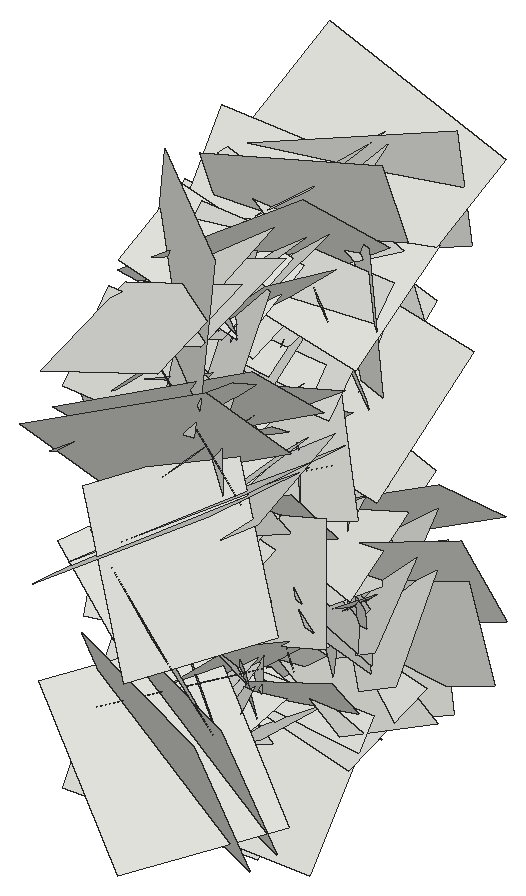
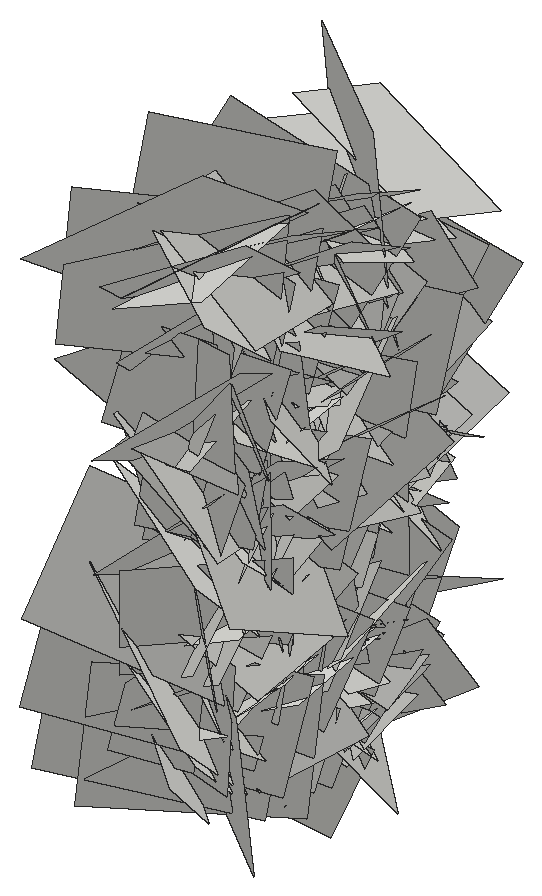
# SketchUp Ruby script. Lengths in inches.
U = 1.inch
M = Sketchup.active_model
def pt(a) = Geom::Point3d.new(a.map { |v| v * U })
def face(e, loops, mat)
  f = e.add_face(loops[0].map { |a| pt(a) })
  loops[1..].each { |l| e.add_face(l.map { |a| pt(a) }).erase! }
  f.material = f.back_material = mat if mat
  f
end
# faces: each face lists its corners as indices into pts; further lists are holes
def faces(e, pts, list, mat = nil) = list.each { |f| face(e, (f[0].is_a?(Array) ? f : [f]).map { |l| l.map { |i| pts[i] } }, mat) }
# xy, xz, yz: faces in a plane at the given z, y or x. An outline is a flat list of corners, or four numbers for a rectangle; further outlines are holes
def ring(l) = l.size == 4 ? [[l[0], l[1]], [l[2], l[1]], [l[2], l[3]], [l[0], l[3]]] : l.each_slice(2).to_a
def flat(e, list, mat, &to3) = list.each { |f| face(e, (f[0].is_a?(Array) ? f : [f]).map { |l| ring(l).map { |u, v| to3.(u, v) } }, mat) }
def xy(e, z, list, mat = nil) = flat(e, list, mat) { |x, y| [x, y, z] }
def xz(e, y, list, mat = nil) = flat(e, list, mat) { |x, z| [x, y, z] }
def yz(e, x, list, mat = nil) = flat(e, list, mat) { |y, z| [x, y, z] }
def lines(e, pts, list) = list.each { |a, b| e.add_line(pt(pts[a]), pt(pts[b])) }
# prism: a flat outline (further loops are holes) pulled along v
def prism(e, loops, v, mat = nil)
  f = face(e, loops, mat); d = Geom::Vector3d.new(v.map { |x| x * U })
  f.pushpull(f.normal.samedirection?(d) ? d.length : -d.length)
end
def box(e, o, s, mat = nil) = prism(e, [[o, [o[0] + s[0], o[1], o[2]], [o[0] + s[0], o[1] + s[1], o[2]], [o[0], o[1] + s[1], o[2]]]], [0, 0, s[2]], mat)
def at(x, y, z, deg = 0) = Geom::Transformation.translation(pt([x, y, z])) * Geom::Transformation.rotation(ORIGIN, Z_AXIS, deg.degrees)
def axes(o, x, y, z) = Geom::Transformation.new([*x, 0, *y, 0, *z, 0, *pt(o).to_a, 1])
def part(name) = M.definitions.add(name)
# library, detail: a bought-in or finely detailed component or shape, given as its bounding box
def library(name, o, s) = part(name).tap { |d| box(d.entities, o, s) }
def detail(e, o, s) = box(e.add_group.entities, o, s)
def put(e, d, t, mat = nil) = e.add_instance(d, t).tap { |i| i.material = mat if mat }
def group(e, t, mat = nil) = e.add_group.tap { |g| g.transformation = t; g.material = mat if mat }.entities
root = M.entities
c1 = part("Component\#6")
p = [[0.01,0,0],[0,3.24,4.54],[4.32,3.24,4.54],[4.33,0,0]]
faces(c1.entities,p,[[0,1,2,3]])
put(root,c1,axes([424.49,133.2,0.29],[0.16868,0.00753,1.30134],[0.16064,1.302,-0.02607],[-1.37005,0.15359,0.15716]))
put(root,c1,axes([420.52,134.57,7.51],[-0.06425,-0.0713,-0.65597],[0.02618,-0.65852,0.06929],[0.69893,0.01811,-0.0629]))
put(root,c1,axes([424.49,128.52,17.74],[-0.08604,0.43028,-0.81229],[-0.04293,-0.81633,-0.42838],[-0.97342,-0.00203,0.0907]))
put(root,c1,axes([420.52,132.11,13.83],[-0.12823,-0.67114,-0.46171],[-0.10246,-0.45164,0.68184],[0.85739,-0.15435,0.01243]))
put(root,c1,axes([424.49,133.79,15.82],[-0.11741,-0.82822,-0.37202],[-0.00882,-0.37384,0.83474],[-0.96237,0.10447,0.03774]))
put(root,c1,axes([420.52,131.53,3.64],[-0.03356,0.34972,-0.55611],[0.01458,-0.55628,-0.35061],[0.69619,0.02851,-0.01946]))
put(root,c1,axes([420.52,130.57,14.69],[-0.08088,0.56373,-0.36339],[0.06437,-0.35843,-0.56878],[0.70803,0.09698,0.0102]))
put(root,c1,axes([424.49,130.125,12.36],[0.14413,1.23778,0.56401],[0.30073,0.52855,-1.22835],[-1.41013,0.23923,-0.20431]))
put(root,c1,axes([424.49,129.28,18.375],[-0.15104,-0.37703,-0.77667],[0.00911,-0.78776,0.38083],[-0.9151,0.05438,0.13199]))
put(root,c1,axes([424.49,132.6,22.9],[-0.05818,0.99288,0.05669],[0.07779,0.06066,-0.99145],[-1.05129,-0.05046,-0.07649]))
put(root,c1,axes([420.52,133.3125,17.59],[0.01529,0.27468,0.5349],[0.08187,0.52978,-0.27413],[0.6321,-0.07526,0.02257]))
put(root,c1,axes([420.52,129.84,16.13],[0.05288,0.68465,0.04631],[-0.09068,0.05228,-0.68068],[0.72171,-0.04359,-0.08892]))
put(root,c1,axes([424.49,129.45,15.69],[0.00555,0.72683,0.86308],[0.19522,0.85097,-0.71774],[-1.18002,0.1442,-0.11468]))
put(root,c1,axes([420.52,129.41,10.95],[-0.18775,-0.48629,-0.69123],[0.00245,-0.70652,0.49646],[0.89586,-0.09998,-0.14623]))
put(root,c1,axes([420.52,132.63,6.14],[-0.10731,0.87556,-0.00554],[-0.12201,-0.01884,-0.87366],[0.92006,0.09962,-0.1165]))
put(root,c1,axes([424.49,133.96,12.5],[-0.03937,0.24323,0.81298],[-0.12274,0.80469,-0.24604],[-0.89109,-0.12158,-0.00203]))
put(root,c1,axes([424.49,127.6,6.32],[-0.09105,0.77875,-0.27248],[-0.08108,-0.28029,-0.77696],[-0.87078,-0.05533,0.10084]))
put(root,c1,axes([424.49,133.1,9.3125],[0.02086,0.87239,-0.16813],[-0.14049,-0.16341,-0.8634],[-0.93122,0.04419,0.12649]))
put(root,c1,axes([424.49,131.05,1.96],[0.03915,-1.05631,0.36623],[0.17317,0.36759,1.04378],[-1.17236,0.01903,0.16641]))
put(root,c1,axes([420.52,133.88,6.93],[-0.12434,-0.60409,0.41763],[0.12699,0.40152,0.61444],[0.76804,-0.16419,-0.03398]))
put(root,c1,axes([424.49,136.93,7.59],[0.11136,0.24127,-0.97313],[-0.07388,-0.97433,-0.24909],[-1.06018,0.09324,-0.08486]))
put(root,c1,axes([420.52,130.03,2.94],[-0.11679,-0.3481,0.76621],[-0.04914,0.77408,0.34502],[0.89071,-0.00294,0.1195]))
put(root,c1,axes([420.52,129.23,5.41],[-0.17398,-0.60139,0.60701],[0.02487,0.6147,0.61536],[0.9054,-0.13245,0.09973]))
put(root,c1,axes([424.49,132.5,3.06],[0.12033,-0.77552,-0.96336],[0.26418,-0.93322,0.78062],[-1.28404,-0.26468,0.07033]))
put(root,c1,axes([420.52,129.18,10.77],[0.08644,0.04023,-0.60323],[0.06997,-0.60565,-0.03147],[0.63702,0.06107,0.08531]))
put(root,c1,axes([424.49,132.55,10.48],[0.11298,-1.07137,-0.22101],[0.09706,-0.21254,1.07447],[-1.1555,-0.12261,0.06864]))
put(root,c1,axes([420.52,128.34,18.92],[0.04874,0.38349,0.62334],[-0.06251,0.62448,-0.37984],[0.77325,0.02631,-0.07]))
put(root,c1,axes([420.52,129.8,15.91],[0.05085,-0.71724,0.33006],[-0.13843,0.31891,0.71198],[0.82538,0.09767,0.09907]))
put(root,c1,axes([424.49,127.86,19.19],[0.25173,1.01088,0.57921],[0.04385,0.58343,-1.03521],[-1.23418,0.22691,0.08136]))
put(root,c1,axes([424.49,127.34,21.1],[0.03089,0.79811,0.32897],[-0.11706,0.3299,-0.79059],[-0.90753,-0.01539,0.11317]))
put(root,c1,axes([420.52,133.42,16.97],[-0.14677,0.94615,0.46149],[-0.22557,0.4307,-0.94687],[1.09283,0.21597,-0.13346]))
put(root,c1,axes([420.52,133.96,6.46],[-0.0893,0.11056,0.97068],[-0.19494,0.95507,-0.12474],[1.01706,0.19277,0.06132]))
put(root,c1,axes([424.49,136.53,11.26],[0.01536,-0.64622,-0.54667],[-0.11065,-0.54394,0.64022],[-0.89037,0.05645,-0.089]))
put(root,c1,axes([420.52,131.99,-0.9375],[0.0225,-0.54484,0.50649],[-0.02225,0.50605,0.54525],[0.78821,0.02984,0.00093]))
put(root,c1,axes([424.49,127.95,5.4],[-0.05879,0.74539,0.22064],[-0.10629,0.21249,-0.74307],[-0.81711,-0.08127,0.08079]))
put(root,c1,axes([420.52,125.86,8.82],[0.02658,0.53015,0.39509],[0.11889,0.38623,-0.52538],[0.69069,-0.08688,0.07523]))
put(root,c1,axes([420.52,131.86,3.01],[0.01467,-0.55248,-0.51034],[-0.00827,-0.51051,0.55244],[0.7972,0.00487,0.01512]))
put(root,c1,axes([420.52,136.82,15.87],[-0.16772,-0.74319,-0.48228],[0.03783,-0.49486,0.75087],[0.93836,-0.11289,-0.11647]))
put(root,c1,axes([424.49,125.93,11.7],[-0.16945,0.67455,-0.05214],[-0.09647,-0.07453,-0.68517],[-0.71064,-0.15073,0.10544]))
put(root,c1,axes([424.49,127.92,4.7],[-0.092,0.70183,0.2556],[-0.07294,0.24871,-0.70628],[-0.78837,-0.10491,0.03552]))
put(root,c1,axes([424.49,128.53,16.93],[0.30517,1.08519,-0.55956],[0.1011,-0.59314,-1.10124],[-1.29027,0.21019,-0.21864]))
put(root,c1,axes([420.52,137.37,4.77],[-0.01509,-0.67708,-0.46908],[-0.05072,-0.46768,0.67651],[0.87164,-0.03894,0.03124]))
put(root,c1,axes([424.49,133.14,16.06],[0.03738,-0.31853,0.81486],[-0.04959,0.81367,0.32009],[-0.92608,-0.05642,0.01575]))
put(root,c1,axes([424.49,133.58,20.74],[0.06025,0.71815,0.57437],[0.00066,0.57544,-0.71955],[-0.97476,0.04478,0.03501]))
put(root,c1,axes([424.49,131.35,15.19],[-0.02447,0.82058,-0.14823],[-0.01236,-0.14859,-0.82075],[-0.8838,-0.02064,0.01558]))
put(root,c1,axes([420.52,130.01,4.69],[0.05447,0.12092,0.77662],[-0.06993,0.77619,-0.11649],[0.83019,0.05744,-0.06077]))
put(root,c1,axes([424.49,135.14,15.06],[0.15738,0.18416,-1.10832],[0.16264,-1.1108,-0.16402],[-1.17977,-0.12857,-0.17046]))
put(root,c1,axes([424.49,133.07,14.74],[0.12706,0.28525,0.91315],[-0.02767,0.92092,-0.28425],[-1.01369,0.01061,0.12222]))
put(root,c1,axes([424.49,132.96,18.89],[0.10145,-0.91774,-0.17179],[-0.02227,-0.17476,0.92192],[-0.98945,-0.09016,-0.03837]))
put(root,c1,axes([420.52,135.65,2.32],[-0.1935,-1.06071,0.09437],[-0.13048,0.11613,1.0671],[1.12123,-0.16954,0.14047]))
put(root,c1,axes([420.52,136.42,13.64],[0.14309,-0.55174,0.41683],[-0.03038,0.41987,0.56505],[0.73236,0.12522,-0.058]))
put(root,c1,axes([424.49,137.27,19.36],[0.1763,0.15017,-0.9005],[-0.15684,-0.89878,-0.17721],[-0.95491,0.17535,-0.13715]))
put(root,c1,axes([424.49,130.2,1.79],[0.1042,-0.77086,0.73803],[0.17604,0.74317,0.75412],[-1.11745,0.04519,0.18762]))
put(root,c1,axes([424.49,136.01,11.51],[-0.06598,-0.27091,0.62957],[-0.16839,0.62065,0.25136],[-0.70672,-0.12259,-0.11867]))
put(root,c1,axes([420.52,133.51,8.98],[-0.15319,0.47062,-0.90401],[-0.09722,-0.91536,-0.46187],[1.07594,-0.0157,-0.17044]))
put(root,c1,axes([424.49,126.24,11.02],[-0.17433,0.41563,0.4957],[-0.04437,0.50356,-0.43611],[-0.68427,-0.13854,-0.09801]))
put(root,c1,axes([420.52,132.67,11.61],[-0.16439,-1.14375,-0.17253],[-0.24163,-0.14044,1.13591],[1.20204,-0.18465,0.20475]))
put(root,c1,axes([424.49,132.67,11.61],[0.16439,-1.14375,-0.17253],[0.24163,-0.14044,1.13591],[-1.20204,-0.18465,0.20475]))
put(root,c1,axes([420.52,126.24,11.02],[0.17433,0.41563,0.4957],[0.04437,0.50356,-0.43611],[0.68427,-0.13854,-0.09801]))
put(root,c1,axes([424.49,133.51,8.98],[0.15319,0.47062,-0.90401],[0.09722,-0.91536,-0.46187],[-1.07594,-0.0157,-0.17044]))
put(root,c1,axes([420.52,136.01,11.51],[0.06598,-0.27091,0.62957],[0.16839,0.62065,0.25136],[0.70672,-0.12259,-0.11867]))
put(root,c1,axes([420.52,130.2,1.79],[-0.1042,-0.77086,0.73803],[-0.17604,0.74317,0.75412],[1.11745,0.04519,0.18762]))
put(root,c1,axes([420.52,137.27,19.36],[-0.1763,0.15017,-0.9005],[0.15684,-0.89878,-0.17721],[0.95491,0.17535,-0.13715]))
put(root,c1,axes([424.49,136.42,13.64],[-0.14309,-0.55174,0.41683],[0.03038,0.41987,0.56505],[-0.73236,0.12522,-0.058]))
put(root,c1,axes([424.49,135.65,2.32],[0.1935,-1.06071,0.09437],[0.13048,0.11613,1.0671],[-1.12123,-0.16954,0.14047]))
put(root,c1,axes([420.52,132.96,18.89],[-0.10145,-0.91774,-0.17179],[0.02227,-0.17476,0.92192],[0.98945,-0.09016,-0.03837]))
put(root,c1,axes([420.52,133.07,14.74],[-0.12706,0.28525,0.91315],[0.02767,0.92092,-0.28425],[1.01369,0.01061,0.12222]))
put(root,c1,axes([420.52,135.14,15.06],[-0.15738,0.18416,-1.10832],[-0.16264,-1.1108,-0.16402],[1.17977,-0.12857,-0.17046]))
put(root,c1,axes([424.49,130.01,4.69],[-0.05447,0.12092,0.77662],[0.06993,0.77619,-0.11649],[-0.83019,0.05744,-0.06077]))
put(root,c1,axes([420.52,131.35,15.19],[0.02447,0.82058,-0.14823],[0.01236,-0.14859,-0.82075],[0.8838,-0.02064,0.01558]))
put(root,c1,axes([420.52,133.58,20.74],[-0.06025,0.71815,0.57437],[-0.00066,0.57544,-0.71955],[0.97476,0.04478,0.03501]))
put(root,c1,axes([420.52,133.14,16.06],[-0.03738,-0.31853,0.81486],[0.04959,0.81367,0.32009],[0.92608,-0.05642,0.01575]))
put(root,c1,axes([424.49,137.37,4.77],[0.01509,-0.67708,-0.46908],[0.05072,-0.46768,0.67651],[-0.87164,-0.03894,0.03124]))
put(root,c1,axes([420.52,128.53,16.93],[-0.30517,1.08519,-0.55956],[-0.1011,-0.59314,-1.10124],[1.29027,0.21019,-0.21864]))
put(root,c1,axes([420.52,127.92,4.7],[0.092,0.70183,0.2556],[0.07294,0.24871,-0.70628],[0.78837,-0.10491,0.03552]))
put(root,c1,axes([420.52,125.93,11.7],[0.16945,0.67455,-0.05214],[0.09647,-0.07453,-0.68517],[0.71064,-0.15073,0.10544]))
put(root,c1,axes([424.49,136.82,15.87],[0.16772,-0.74319,-0.48228],[-0.03783,-0.49486,0.75087],[-0.93836,-0.11289,-0.11647]))
put(root,c1,axes([424.49,131.86,3.01],[-0.01467,-0.55248,-0.51034],[0.00827,-0.51051,0.55244],[-0.7972,0.00487,0.01512]))
put(root,c1,axes([424.49,125.86,8.82],[-0.02658,0.53015,0.39509],[-0.11889,0.38623,-0.52538],[-0.69069,-0.08688,0.07523]))
put(root,c1,axes([420.52,127.95,5.4],[0.05879,0.74539,0.22064],[0.10629,0.21249,-0.74307],[0.81711,-0.08127,0.08079]))
put(root,c1,axes([424.49,131.99,-0.9375],[-0.0225,-0.54484,0.50649],[0.02225,0.50605,0.54525],[-0.78821,0.02984,0.00093]))
put(root,c1,axes([420.52,136.53,11.26],[-0.01536,-0.64622,-0.54667],[0.11065,-0.54394,0.64022],[0.89037,0.05645,-0.089]))
put(root,c1,axes([424.49,133.96,6.46],[0.0893,0.11056,0.97068],[0.19494,0.95507,-0.12474],[-1.01706,0.19277,0.06132]))
put(root,c1,axes([420.52,127.34,21.1],[-0.03089,0.79811,0.32897],[0.11706,0.3299,-0.79059],[0.90753,-0.01539,0.11317]))
put(root,c1,axes([420.52,127.86,19.19],[-0.25173,1.01088,0.57921],[-0.04385,0.58343,-1.03521],[1.23418,0.22691,0.08136]))
put(root,c1,axes([424.49,129.8,15.91],[-0.05085,-0.71724,0.33006],[0.13843,0.31891,0.71198],[-0.82538,0.09767,0.09907]))
put(root,c1,axes([424.49,128.34,18.92],[-0.04874,0.38349,0.62334],[0.06251,0.62448,-0.37984],[-0.77325,0.02631,-0.07]))
put(root,c1,axes([420.52,132.55,10.48],[-0.11298,-1.07137,-0.22101],[-0.09706,-0.21254,1.07447],[1.1555,-0.12261,0.06864]))
put(root,c1,axes([424.49,129.18,10.77],[-0.08644,0.04023,-0.60323],[-0.06997,-0.60565,-0.03147],[-0.63702,0.06107,0.08531]))
put(root,c1,axes([420.52,132.5,3.06],[-0.12033,-0.77552,-0.96336],[-0.26418,-0.93322,0.78062],[1.28404,-0.26468,0.07033]))
put(root,c1,axes([424.49,129.23,5.41],[0.17398,-0.60139,0.60701],[-0.02487,0.6147,0.61536],[-0.9054,-0.13245,0.09973]))
put(root,c1,axes([424.49,130.03,2.94],[0.11679,-0.3481,0.76621],[0.04914,0.77408,0.34502],[-0.89071,-0.00294,0.1195]))
put(root,c1,axes([420.52,136.93,7.59],[-0.11136,0.24127,-0.97313],[0.07388,-0.97433,-0.24909],[1.06018,0.09324,-0.08486]))
put(root,c1,axes([424.49,133.88,6.93],[0.12434,-0.60409,0.41763],[-0.12699,0.40152,0.61444],[-0.76804,-0.16419,-0.03398]))
put(root,c1,axes([420.52,131.05,1.96],[-0.03915,-1.05631,0.36623],[-0.17317,0.36759,1.04378],[1.17236,0.01903,0.16641]))
put(root,c1,axes([420.52,133.1,9.3125],[-0.02086,0.87239,-0.16813],[0.14049,-0.16341,-0.8634],[0.93122,0.04419,0.12649]))
put(root,c1,axes([420.52,127.6,6.32],[0.09105,0.77875,-0.27248],[0.08108,-0.28029,-0.77696],[0.87078,-0.05533,0.10084]))
put(root,c1,axes([420.52,133.96,12.5],[0.03937,0.24323,0.81298],[0.12274,0.80469,-0.24604],[0.89109,-0.12158,-0.00203]))
put(root,c1,axes([424.49,132.63,6.14],[0.10731,0.87556,-0.00554],[0.12201,-0.01884,-0.87366],[-0.92006,0.09962,-0.1165]))
put(root,c1,axes([424.49,129.41,10.95],[0.18775,-0.48629,-0.69123],[-0.00245,-0.70652,0.49646],[-0.89586,-0.09998,-0.14623]))
put(root,c1,axes([420.52,129.45,15.69],[-0.00555,0.72683,0.86308],[-0.19522,0.85097,-0.71774],[1.18002,0.1442,-0.11468]))
put(root,c1,axes([424.49,129.84,16.13],[-0.05288,0.68465,0.04631],[0.09068,0.05228,-0.68068],[-0.72171,-0.04359,-0.08892]))
put(root,c1,axes([424.49,133.3125,17.59],[-0.01529,0.27468,0.5349],[-0.08187,0.52978,-0.27413],[-0.6321,-0.07526,0.02257]))
put(root,c1,axes([420.52,132.6,22.9],[0.05818,0.99288,0.05669],[-0.07779,0.06066,-0.99145],[1.05129,-0.05046,-0.07649]))
put(root,c1,axes([420.52,129.28,18.375],[0.15104,-0.37703,-0.77667],[-0.00911,-0.78776,0.38083],[0.9151,0.05438,0.13199]))
put(root,c1,axes([420.52,130.125,12.36],[-0.14413,1.23778,0.56401],[-0.30073,0.52855,-1.22835],[1.41013,0.23923,-0.20431]))
put(root,c1,axes([424.49,130.57,14.69],[0.08088,0.56373,-0.36339],[-0.06437,-0.35843,-0.56878],[-0.70803,0.09698,0.0102]))
put(root,c1,axes([424.49,131.53,3.64],[0.03356,0.34972,-0.55611],[-0.01458,-0.55628,-0.35061],[-0.69619,0.02851,-0.01946]))
put(root,c1,axes([420.52,133.79,15.82],[0.11741,-0.82822,-0.37202],[0.00882,-0.37384,0.83474],[0.96237,0.10447,0.03774]))
put(root,c1,axes([424.49,132.11,13.83],[0.12823,-0.67114,-0.46171],[0.10246,-0.45164,0.68184],[-0.85739,-0.15435,0.01243]))
put(root,c1,axes([420.52,128.52,17.74],[0.08604,0.43028,-0.81229],[0.04293,-0.81633,-0.42838],[0.97342,-0.00203,0.0907]))
put(root,c1,axes([424.49,134.57,7.51],[0.06425,-0.0713,-0.65597],[-0.02618,-0.65852,0.06929],[-0.69893,0.01811,-0.0629]))
put(root,c1,axes([420.52,133.2,0.29],[-0.16868,0.00753,1.30134],[-0.16064,1.302,-0.02607],[1.37005,0.15359,0.15716]))
put(root,c1,axes([424.49,127.28,0.51],[0.04452,-0.40985,0.5808],[0.07759,0.58122,0.40485],[-0.7495,0.03582,0.07641]))
put(root,c1,axes([420.52,129.68,16.21],[0.16446,-0.17941,-0.82447],[0.07006,-0.83314,0.19373],[0.89165,0.09856,0.13685]))
put(root,c1,axes([424.49,134.26,15.51],[0.13639,0.72841,-0.25059],[0.07067,-0.26364,-0.7321],[-0.81346,0.09922,-0.10562]))
put(root,c1,axes([420.52,128.87,2.92],[0.01411,0.95221,-0.19006],[0.11482,-0.19035,-0.94606],[1.02282,0.00823,0.10882]))
put(root,c1,axes([420.52,138.97,11.375],[-0.02639,-0.72989,-0.72722],[0.07911,-0.7268,0.72691],[1.08928,0.0351,-0.07041]))
put(root,c1,axes([420.52,131.74,20.5625],[-0.11289,-0.41624,-1.03402],[0.06809,-1.03929,0.41174],[1.17957,0.02016,-0.12272]))
put(root,c1,axes([424.49,131.9,7.66],[0.03371,0.19161,0.61883],[0.06203,0.6162,-0.1938],[-0.68388,0.06533,0.01292]))
put(root,c1,axes([420.52,134.95,12.42],[0.03363,0.92541,-1.00089],[-0.39451,-0.95725,-0.89685],[1.39004,-0.29406,-0.23032]))
put(root,c1,axes([424.49,131.8,8.64],[0.08497,0.05507,0.67491],[0.04101,0.67814,-0.05993],[-0.71661,0.04534,0.0766]))
put(root,c1,axes([420.52,137.87,11.82],[0.23548,-0.98581,-0.19043],[-0.17104,-0.22756,0.98976],[1.05044,0.18394,0.20385]))
put(root,c1,axes([420.52,129.625,19.87],[-0.14331,0.9196,0.97349],[-0.15794,0.96203,-0.92947],[1.41069,0.20113,-0.00516]))
put(root,c1,axes([420.52,130.99,8.6],[0.04494,-0.64922,0.68663],[0.20873,0.6783,0.62918],[0.97967,-0.11474,-0.16555]))
put(root,c1,axes([420.52,133.91,11.1875],[-0.02059,0.92356,-0.8814],[-0.20413,-0.87353,-0.91107],[1.33776,-0.11908,-0.15259]))
put(root,c1,axes([420.52,128.56,10.3125],[-0.23413,0.04823,1.24691],[0.1221,1.26168,-0.02839],[1.31707,-0.10839,0.22429]))
put(root,c1,axes([420.52,131.94,16.85],[-0.08825,-0.96476,0.81898],[-0.08011,0.82307,0.9619],[1.33903,-0.01434,0.11152]))
put(root,c1,axes([420.52,131.18,15.16],[0.15294,-1.16278,0.39158],[-0.28955,0.35393,1.15166],[1.26792,0.22109,0.21577]))
put(root,c1,axes([424.49,134.77,2.57],[0.05447,0.40704,0.46107],[0.08155,0.45478,-0.41007],[-0.64681,0.09162,-0.01288]))
put(root,c1,axes([420.52,134.14,22.88],[0.03825,0.99518,-0.25742],[0.13842,-0.25993,-0.98657],[1.08078,-0.00193,0.13547]))
put(root,c1,axes([419.8,124.93,11.12],[0.54058,0.75668,0.32998],[0.30141,0.20311,-0.90522],[0.82148,-0.57246,0.11499]))
put(root,c1,axes([420.52,127.92,6.47],[-0.03611,0.05394,1.13531],[0.09971,1.13206,-0.05096],[1.20066,-0.09239,0.03838]))
put(root,c1,axes([424.49,138.1,17.99],[0.00934,-0.49027,-0.41508],[0.1892,-0.3969,0.47259],[-0.65411,-0.1218,0.13076]))
put(root,c1,axes([420.52,127.69,20.12],[-0.02742,-1.01137,-0.35231],[0.21232,-0.35076,0.99222],[1.1152,0.04191,-0.19757]))
put(root,c1,axes([420.52,130,20.12],[-0.02742,-1.01137,-0.35231],[0.21232,-0.35076,0.99222],[1.1152,0.04191,-0.19757]))
put(root,c1,axes([424.49,129.35,18.22],[0.07955,-0.40219,0.442],[0.06566,0.44831,0.39741],[-0.63004,-0.00406,0.09723]))
put(root,c1,axes([420.52,129.81,24.32],[-0.08615,-0.07511,-1.33483],[-0.12267,-1.33188,0.08199],[1.41184,-0.12031,-0.07433]))
put(root,c1,axes([420.52,131.16,1.32],[0.11103,-1.00768,0.14491],[0.13016,0.15712,1.00381],[1.07125,0.08535,-0.13699]))
put(root,c1,axes([420.52,136.29,19.65],[0.239,0.33681,-1.04778],[-0.13934,-1.05364,-0.36698],[1.15826,-0.19625,0.17205]))
put(root,c1,axes([420.52,129.42,5.47],[-0.26825,1.30607,0.06413],[0.25565,0.11082,-1.30519],[1.36232,0.23638,0.25756]))
put(root,c1,axes([420.52,126.61,12.8],[-0.1414,-0.87971,0.87765],[0.19082,0.8597,0.88908],[1.30331,-0.22132,-0.03495]))
put(root,c1,axes([420.52,133.96,9.66],[0.06967,-1.04066,0.34132],[0.1454,0.34706,1.03175],[1.15177,0.01914,-0.15089]))
put(root,c1,axes([420.52,134.94,17.85],[0.08672,-0.29938,1.1859],[-0.04442,1.18717,0.30259],[1.29573,0.06074,-0.069]))
put(root,c1,axes([420.52,129.48,20.64],[-0.14207,1.22324,0.51937],[0.11373,0.53026,-1.2212],[1.40407,0.08082,0.15147]))
put(root,c1,axes([420.52,129.66,12.47],[-0.1081,-1.2535,0.58167],[-0.00417,0.58351,1.25678],[1.46479,-0.09085,0.0465]))
put(root,c1,axes([420.52,125.82,11.42],[0.20547,0.4933,-0.99975],[0.03886,-1.01702,-0.49472],[1.18108,-0.05236,0.1902]))
put(root,c1,axes([420.52,131.95,0.87],[0.07095,-0.70744,0.83659],[0.30432,0.82019,0.6706],[1.12076,-0.17792,-0.23504]))
put(root,c1,axes([420.52,139.8125,5.82],[0.12038,-0.94885,-0.86303],[-0.08352,-0.86993,0.94607],[1.35702,0.03063,0.13479]))
put(root,c1,axes([420.52,133.04,19.75],[0.14526,-0.49923,0.95494],[0.24012,0.95446,0.46647],[1.11669,-0.1403,-0.22453]))
put(root,c1,axes([420.52,128.24,17.68],[0.22785,0.52614,1.07761],[-0.06777,1.09826,-0.52347],[1.26934,-0.03581,-0.22138]))
put(root,c1,axes([420.52,133.15,22.79],[0.15509,1.06813,0.73269],[-0.10614,0.74447,-1.06531],[1.36888,-0.06329,-0.16562]))
put(root,c1,axes([420.52,132.12,7.08],[-0.00585,1.22451,-0.43101],[0.11167,-0.42917,-1.22063],[1.3715,0.04016,0.09755]))
put(root,c1,axes([420.52,125.99,1.35],[0.00241,0.79041,1.08039],[0.06651,1.07914,-0.78963],[1.41741,-0.05198,0.03522]))
put(root,c1,axes([420.52,127.67,13.74],[0.06329,-0.97705,0.81505],[0.12838,0.8166,0.97005],[1.34259,-0.03203,-0.13118]))
put(root,c1,axes([420.52,137,19.49],[0.23927,-0.1296,-1.18474],[0.04055,-1.20439,0.13904],[1.26266,0.06324,0.22004]))
put(root,c1,axes([420.52,135.39,1.18],[0.01455,-0.40823,1.27358],[0.1801,1.26386,0.40328],[1.40617,-0.15765,-0.06483]))
put(root,c1,axes([420.52,128.0625,10.23],[0.10909,-1.3698,0.20566],[-0.00727,0.20572,1.37363],[1.46824,0.1028,-0.00848]))
put(root,c1,axes([420.52,129.98,10.23],[0.10909,-1.3698,0.20566],[-0.00727,0.20572,1.37363],[1.46824,0.1028,-0.00848]))
put(root,c1,axes([420.52,138.98,4.78],[0.22268,-0.9196,-0.8307],[0.07298,-0.83259,0.9391],[1.31157,0.20246,0.08879]))
put(root,c1,axes([419.35,124.5,5.79],[0.83668,1.07369,0.2523],[0.21003,0.16716,-1.33127],[1.15009,-0.81162,0.05958]))
put(root,c1,axes([420.52,130.78,10.54],[0.24762,-1.26357,-0.1726],[-0.00687,-0.17664,1.28442],[1.3518,0.23056,0.03815]))
put(root,c1,axes([420.52,136.82,5.83],[0.1656,-1.02965,0.80161],[0.14776,0.81588,1.02082],[1.37528,0.03632,-0.2062]))
put(root,c1,axes([420.52,130.15,15.41],[0.24379,0.89731,1.03665],[0.02149,1.04879,-0.91232],[1.45316,-0.16605,-0.16042]))
put(root,c1,axes([420.52,135.96,3.29],[0.1622,-0.76384,1.11136],[0.23079,1.11781,0.7383],[1.4107,-0.09505,-0.24857]))
put(root,c1,axes([420.52,125.3125,7.6875],[0.15543,0.49215,-1.26812],[0.29157,-1.25984,-0.45713],[1.41209,0.20597,0.23397]))
put(root,c1,axes([420.52,126.76,7.6875],[0.15543,0.49215,-1.26812],[0.29157,-1.25984,-0.45713],[1.41209,0.20597,0.23397]))
put(root,c1,axes([420.41,125.5,13.2],[1.07209,0.56535,0.5401],[0.40295,0.41611,-1.14744],[0.72423,-1.06841,-0.1611]))
